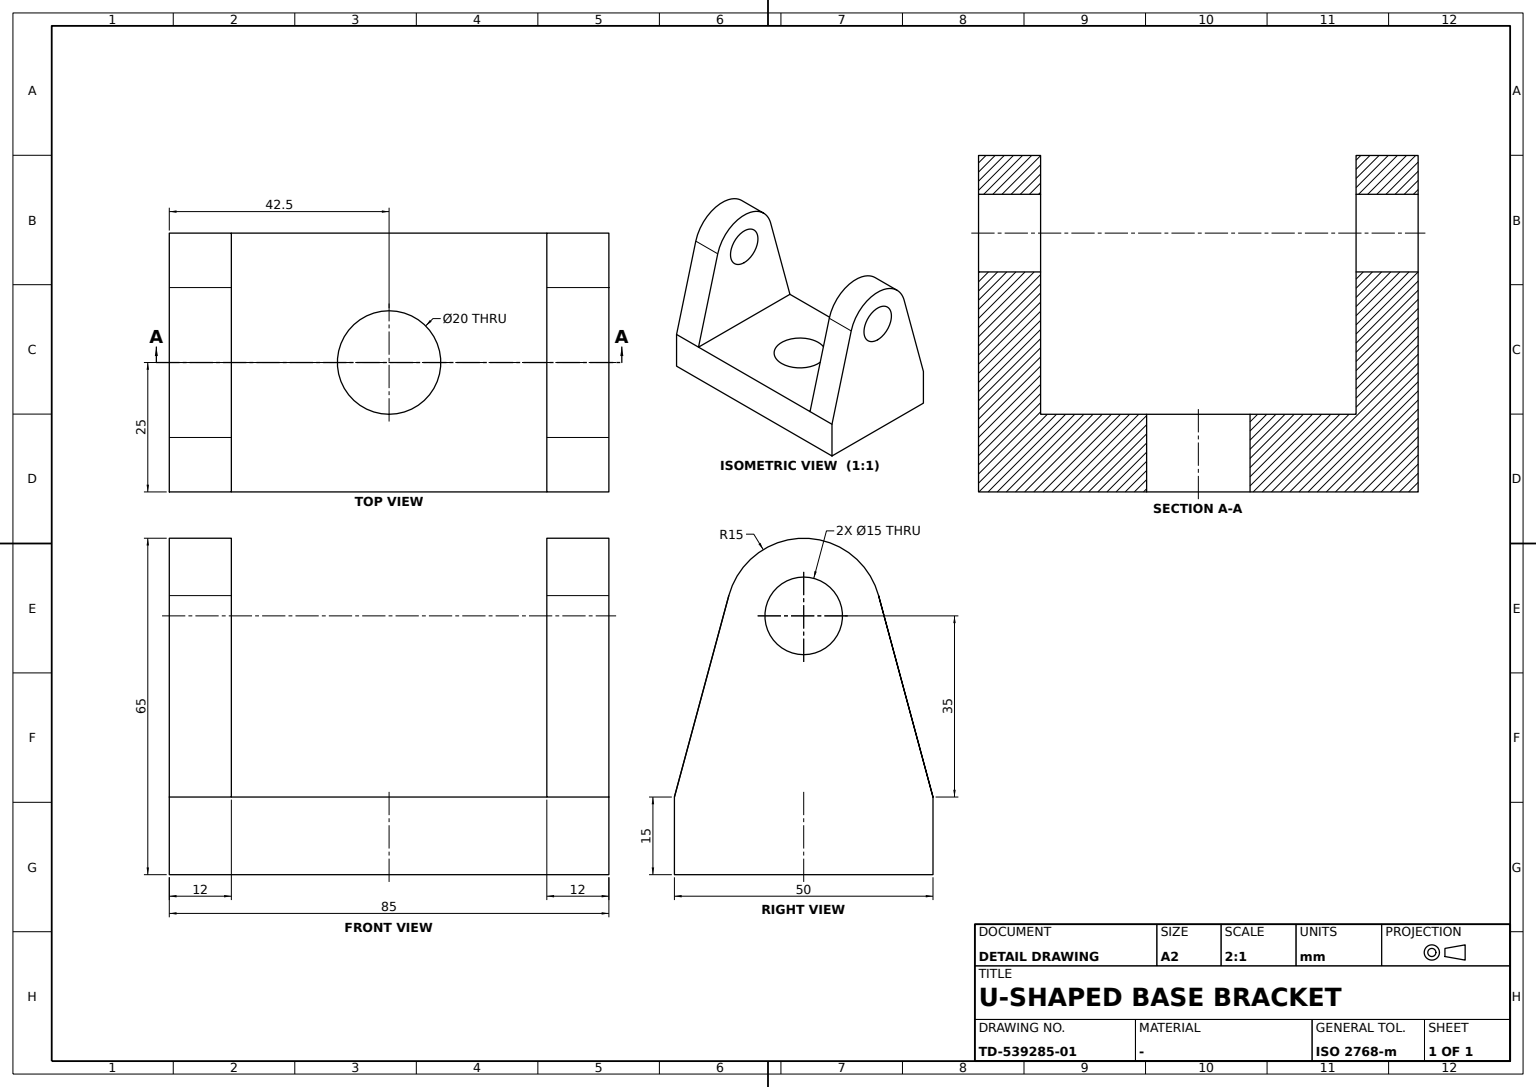
ISO-10303-21;
HEADER;
FILE_DESCRIPTION((''),'2;1');
FILE_NAME('','',(''),(''),'','','');
FILE_SCHEMA(('AUTOMOTIVE_DESIGN'));
ENDSEC;
DATA;
#1=APPLICATION_CONTEXT('');
#2=PRODUCT_CONTEXT('',#1,'mechanical');
#3=PRODUCT('','','',(#2));
#4=PRODUCT_DEFINITION_FORMATION('','',#3);
#5=PRODUCT_DEFINITION_CONTEXT('',#1,'design');
#6=PRODUCT_DEFINITION('','',#4,#5);
#7=PRODUCT_DEFINITION_SHAPE('','',#6);
#8=(LENGTH_UNIT()NAMED_UNIT(*)SI_UNIT(.MILLI.,.METRE.));
#9=(NAMED_UNIT(*)PLANE_ANGLE_UNIT()SI_UNIT($,.RADIAN.));
#10=(NAMED_UNIT(*)SI_UNIT($,.STERADIAN.)SOLID_ANGLE_UNIT());
#11=UNCERTAINTY_MEASURE_WITH_UNIT(LENGTH_MEASURE(0.005),#8,'distance_accuracy_value','');
#12=(GEOMETRIC_REPRESENTATION_CONTEXT(3)GLOBAL_UNCERTAINTY_ASSIGNED_CONTEXT((#11))GLOBAL_UNIT_ASSIGNED_CONTEXT((#8,#9,#10))REPRESENTATION_CONTEXT('',''));
#13=CARTESIAN_POINT('',(-14.480231,-42.5,53.91445));
#14=VERTEX_POINT('',#13);
#15=CARTESIAN_POINT('',(-14.480231,-30.5,53.91445));
#16=VERTEX_POINT('',#15);
#17=CARTESIAN_POINT('',(-14.480231,-36.5,53.91445));
#18=DIRECTION('',(0.,-1.,0.));
#19=VECTOR('',#18,1000.);
#20=LINE('',#17,#19);
#21=EDGE_CURVE('',#14,#16,#20,.F.);
#22=ORIENTED_EDGE('',*,*,#21,.T.);
#23=CARTESIAN_POINT('',(-25.,-30.5,15.));
#24=VERTEX_POINT('',#23);
#25=DIRECTION('',(-0.260963361,0.,-0.965348706));
#26=VECTOR('',#25,1000.);
#27=LINE('',#15,#26);
#28=EDGE_CURVE('',#16,#24,#27,.T.);
#29=ORIENTED_EDGE('',*,*,#28,.T.);
#30=CARTESIAN_POINT('',(-25.,-42.5,15.));
#31=VERTEX_POINT('',#30);
#32=DIRECTION('',(0.,1.,0.));
#33=VECTOR('',#32,1000.);
#34=LINE('',#30,#33);
#35=EDGE_CURVE('',#31,#24,#34,.T.);
#36=ORIENTED_EDGE('',*,*,#35,.F.);
#37=LINE('',#13,#26);
#38=EDGE_CURVE('',#14,#31,#37,.T.);
#39=ORIENTED_EDGE('',*,*,#38,.F.);
#40=EDGE_LOOP('',(#22,#29,#36,#39));
#41=FACE_BOUND('',#40,.T.);
#42=DIRECTION('',(0.965348706,0.,-0.260963361));
#43=AXIS2_PLACEMENT_3D('',#13,#42,#25);
#44=PLANE('',#43);
#45=ADVANCED_FACE('',(#41),#44,.F.);
#46=CARTESIAN_POINT('',(25.,30.5,15.));
#47=VERTEX_POINT('',#46);
#48=CARTESIAN_POINT('',(14.480231,30.5,53.91445));
#49=VERTEX_POINT('',#48);
#50=DIRECTION('',(-0.260963361,0.,0.965348706));
#51=VECTOR('',#50,1000.);
#52=LINE('',#46,#51);
#53=EDGE_CURVE('',#47,#49,#52,.T.);
#54=ORIENTED_EDGE('',*,*,#53,.T.);
#55=CARTESIAN_POINT('',(-14.480231,30.5,53.91445));
#56=VERTEX_POINT('',#55);
#57=CARTESIAN_POINT('',(0.,30.5,50.));
#58=DIRECTION('',(0.,0.,-1.));
#59=AXIS2_PLACEMENT_3D('',#57,#18,#58);
#60=CIRCLE('',#59,15.);
#61=EDGE_CURVE('',#49,#56,#60,.T.);
#62=ORIENTED_EDGE('',*,*,#61,.T.);
#63=CARTESIAN_POINT('',(-25.,30.5,15.));
#64=VERTEX_POINT('',#63);
#65=LINE('',#55,#26);
#66=EDGE_CURVE('',#56,#64,#65,.T.);
#67=ORIENTED_EDGE('',*,*,#66,.T.);
#68=CARTESIAN_POINT('',(0.,30.5,15.));
#69=DIRECTION('',(1.,0.,0.));
#70=VECTOR('',#69,1000.);
#71=LINE('',#68,#70);
#72=EDGE_CURVE('',#64,#47,#71,.T.);
#73=ORIENTED_EDGE('',*,*,#72,.T.);
#74=EDGE_LOOP('',(#54,#62,#67,#73));
#75=FACE_BOUND('',#74,.T.);
#76=CARTESIAN_POINT('',(0.,30.5,42.5));
#77=VERTEX_POINT('',#76);
#78=CIRCLE('',#59,7.5);
#79=EDGE_CURVE('',#77,#77,#78,.T.);
#80=ORIENTED_EDGE('',*,*,#79,.F.);
#81=EDGE_LOOP('',(#80));
#82=FACE_BOUND('',#81,.T.);
#83=CARTESIAN_POINT('',(0.,30.5,0.));
#84=AXIS2_PLACEMENT_3D('',#83,#18,#69);
#85=PLANE('',#84);
#86=ADVANCED_FACE('',(#75,#82),#85,.T.);
#87=CARTESIAN_POINT('',(25.,-30.5,15.));
#88=VERTEX_POINT('',#87);
#89=CARTESIAN_POINT('',(14.480231,-30.5,53.91445));
#90=VERTEX_POINT('',#89);
#91=LINE('',#87,#51);
#92=EDGE_CURVE('',#88,#90,#91,.T.);
#93=ORIENTED_EDGE('',*,*,#92,.F.);
#94=CARTESIAN_POINT('',(0.,-30.5,15.));
#95=LINE('',#94,#70);
#96=EDGE_CURVE('',#24,#88,#95,.T.);
#97=ORIENTED_EDGE('',*,*,#96,.F.);
#98=ORIENTED_EDGE('',*,*,#28,.F.);
#99=CARTESIAN_POINT('',(0.,-30.5,50.));
#100=AXIS2_PLACEMENT_3D('',#99,#18,#58);
#101=CIRCLE('',#100,15.);
#102=EDGE_CURVE('',#90,#16,#101,.T.);
#103=ORIENTED_EDGE('',*,*,#102,.F.);
#104=EDGE_LOOP('',(#93,#97,#98,#103));
#105=FACE_BOUND('',#104,.T.);
#106=CARTESIAN_POINT('',(0.,-30.5,42.5));
#107=VERTEX_POINT('',#106);
#108=CIRCLE('',#100,7.5);
#109=EDGE_CURVE('',#107,#107,#108,.T.);
#110=ORIENTED_EDGE('',*,*,#109,.T.);
#111=EDGE_LOOP('',(#110));
#112=FACE_BOUND('',#111,.T.);
#113=CARTESIAN_POINT('',(0.,-30.5,0.));
#114=AXIS2_PLACEMENT_3D('',#113,#18,#69);
#115=PLANE('',#114);
#116=ADVANCED_FACE('',(#105,#112),#115,.F.);
#117=CARTESIAN_POINT('',(-14.480231,42.5,53.91445));
#118=VERTEX_POINT('',#117);
#119=CARTESIAN_POINT('',(-25.,42.5,15.));
#120=VERTEX_POINT('',#119);
#121=LINE('',#117,#26);
#122=EDGE_CURVE('',#118,#120,#121,.T.);
#123=ORIENTED_EDGE('',*,*,#122,.T.);
#124=EDGE_CURVE('',#64,#120,#34,.T.);
#125=ORIENTED_EDGE('',*,*,#124,.F.);
#126=ORIENTED_EDGE('',*,*,#66,.F.);
#127=EDGE_CURVE('',#56,#118,#20,.F.);
#128=ORIENTED_EDGE('',*,*,#127,.T.);
#129=EDGE_LOOP('',(#123,#125,#126,#128));
#130=FACE_BOUND('',#129,.T.);
#131=ADVANCED_FACE('',(#130),#44,.F.);
#132=CARTESIAN_POINT('',(0.,-42.5,42.5));
#133=VERTEX_POINT('',#132);
#134=CARTESIAN_POINT('',(0.,-42.5,50.));
#135=AXIS2_PLACEMENT_3D('',#134,#18,#58);
#136=CIRCLE('',#135,7.5);
#137=EDGE_CURVE('',#133,#133,#136,.T.);
#138=ORIENTED_EDGE('',*,*,#137,.F.);
#139=EDGE_LOOP('',(#138));
#140=FACE_BOUND('',#139,.T.);
#141=CARTESIAN_POINT('',(25.,-42.5,15.));
#142=VERTEX_POINT('',#141);
#143=CARTESIAN_POINT('',(14.480231,-42.5,53.91445));
#144=VERTEX_POINT('',#143);
#145=LINE('',#141,#51);
#146=EDGE_CURVE('',#142,#144,#145,.T.);
#147=ORIENTED_EDGE('',*,*,#146,.T.);
#148=CIRCLE('',#135,15.);
#149=EDGE_CURVE('',#144,#14,#148,.T.);
#150=ORIENTED_EDGE('',*,*,#149,.T.);
#151=ORIENTED_EDGE('',*,*,#38,.T.);
#152=CARTESIAN_POINT('',(-25.,-42.5,0.));
#153=VERTEX_POINT('',#152);
#154=DIRECTION('',(0.,0.,1.));
#155=VECTOR('',#154,1000.);
#156=LINE('',#152,#155);
#157=EDGE_CURVE('',#153,#31,#156,.T.);
#158=ORIENTED_EDGE('',*,*,#157,.F.);
#159=CARTESIAN_POINT('',(25.,-42.5,0.));
#160=VERTEX_POINT('',#159);
#161=CARTESIAN_POINT('',(0.,-42.5,0.));
#162=LINE('',#161,#70);
#163=EDGE_CURVE('',#153,#160,#162,.T.);
#164=ORIENTED_EDGE('',*,*,#163,.T.);
#165=LINE('',#159,#155);
#166=EDGE_CURVE('',#160,#142,#165,.T.);
#167=ORIENTED_EDGE('',*,*,#166,.T.);
#168=EDGE_LOOP('',(#147,#150,#151,#158,#164,#167));
#169=FACE_BOUND('',#168,.T.);
#170=AXIS2_PLACEMENT_3D('',#152,#18,#69);
#171=PLANE('',#170);
#172=ADVANCED_FACE('',(#140,#169),#171,.T.);
#173=ORIENTED_EDGE('',*,*,#127,.F.);
#174=ORIENTED_EDGE('',*,*,#61,.F.);
#175=CARTESIAN_POINT('',(14.480231,42.5,53.91445));
#176=VERTEX_POINT('',#175);
#177=CARTESIAN_POINT('',(14.480231,-36.5,53.91445));
#178=LINE('',#177,#19);
#179=EDGE_CURVE('',#49,#176,#178,.F.);
#180=ORIENTED_EDGE('',*,*,#179,.T.);
#181=CARTESIAN_POINT('',(0.,42.5,50.));
#182=AXIS2_PLACEMENT_3D('',#181,#18,#58);
#183=CIRCLE('',#182,15.);
#184=EDGE_CURVE('',#176,#118,#183,.T.);
#185=ORIENTED_EDGE('',*,*,#184,.T.);
#186=EDGE_LOOP('',(#173,#174,#180,#185));
#187=FACE_BOUND('',#186,.T.);
#188=CARTESIAN_POINT('',(0.,-36.5,50.));
#189=AXIS2_PLACEMENT_3D('',#188,#18,#69);
#190=CYLINDRICAL_SURFACE('',#189,15.);
#191=ADVANCED_FACE('',(#187),#190,.T.);
#192=ORIENTED_EDGE('',*,*,#92,.T.);
#193=EDGE_CURVE('',#144,#90,#178,.F.);
#194=ORIENTED_EDGE('',*,*,#193,.F.);
#195=ORIENTED_EDGE('',*,*,#146,.F.);
#196=LINE('',#141,#33);
#197=EDGE_CURVE('',#142,#88,#196,.T.);
#198=ORIENTED_EDGE('',*,*,#197,.T.);
#199=EDGE_LOOP('',(#192,#194,#195,#198));
#200=FACE_BOUND('',#199,.T.);
#201=DIRECTION('',(-0.965348706,0.,-0.260963361));
#202=AXIS2_PLACEMENT_3D('',#141,#201,#50);
#203=PLANE('',#202);
#204=ADVANCED_FACE('',(#200),#203,.F.);
#205=CARTESIAN_POINT('',(-25.,0.,15.));
#206=LINE('',#205,#33);
#207=EDGE_CURVE('',#24,#64,#206,.T.);
#208=ORIENTED_EDGE('',*,*,#207,.F.);
#209=ORIENTED_EDGE('',*,*,#96,.T.);
#210=CARTESIAN_POINT('',(25.,0.,15.));
#211=LINE('',#210,#19);
#212=EDGE_CURVE('',#47,#88,#211,.T.);
#213=ORIENTED_EDGE('',*,*,#212,.F.);
#214=ORIENTED_EDGE('',*,*,#72,.F.);
#215=EDGE_LOOP('',(#208,#209,#213,#214));
#216=FACE_BOUND('',#215,.T.);
#217=CARTESIAN_POINT('',(10.,0.,15.));
#218=VERTEX_POINT('',#217);
#219=CARTESIAN_POINT('',(0.,0.,15.));
#220=AXIS2_PLACEMENT_3D('',#219,#154,#69);
#221=CIRCLE('',#220,10.);
#222=EDGE_CURVE('',#218,#218,#221,.T.);
#223=ORIENTED_EDGE('',*,*,#222,.F.);
#224=EDGE_LOOP('',(#223));
#225=FACE_BOUND('',#224,.T.);
#226=AXIS2_PLACEMENT_3D('',#219,#154,#32);
#227=PLANE('',#226);
#228=ADVANCED_FACE('',(#216,#225),#227,.T.);
#229=CARTESIAN_POINT('',(10.,0.,0.));
#230=VERTEX_POINT('',#229);
#231=CARTESIAN_POINT('',(0.,0.,0.));
#232=AXIS2_PLACEMENT_3D('',#231,#154,#69);
#233=CIRCLE('',#232,10.);
#234=EDGE_CURVE('',#230,#230,#233,.T.);
#235=ORIENTED_EDGE('',*,*,#234,.F.);
#236=EDGE_LOOP('',(#235));
#237=FACE_BOUND('',#236,.T.);
#238=ORIENTED_EDGE('',*,*,#222,.T.);
#239=EDGE_LOOP('',(#238));
#240=FACE_BOUND('',#239,.T.);
#241=CARTESIAN_POINT('',(0.,0.,7.5));
#242=AXIS2_PLACEMENT_3D('',#241,#154,#32);
#243=CYLINDRICAL_SURFACE('',#242,10.);
#244=ADVANCED_FACE('',(#237,#240),#243,.F.);
#245=ORIENTED_EDGE('',*,*,#79,.T.);
#246=EDGE_LOOP('',(#245));
#247=FACE_BOUND('',#246,.T.);
#248=CARTESIAN_POINT('',(0.,42.5,42.5));
#249=VERTEX_POINT('',#248);
#250=CIRCLE('',#182,7.5);
#251=EDGE_CURVE('',#249,#249,#250,.T.);
#252=ORIENTED_EDGE('',*,*,#251,.F.);
#253=EDGE_LOOP('',(#252));
#254=FACE_BOUND('',#253,.T.);
#255=CYLINDRICAL_SURFACE('',#189,7.5);
#256=ADVANCED_FACE('',(#247,#254),#255,.F.);
#257=CARTESIAN_POINT('',(25.,42.5,0.));
#258=VERTEX_POINT('',#257);
#259=CARTESIAN_POINT('',(25.,0.,0.));
#260=LINE('',#259,#19);
#261=EDGE_CURVE('',#258,#160,#260,.T.);
#262=ORIENTED_EDGE('',*,*,#261,.T.);
#263=ORIENTED_EDGE('',*,*,#163,.F.);
#264=CARTESIAN_POINT('',(-25.,42.5,0.));
#265=VERTEX_POINT('',#264);
#266=CARTESIAN_POINT('',(-25.,0.,0.));
#267=LINE('',#266,#33);
#268=EDGE_CURVE('',#153,#265,#267,.T.);
#269=ORIENTED_EDGE('',*,*,#268,.T.);
#270=DIRECTION('',(-1.,0.,0.));
#271=VECTOR('',#270,1000.);
#272=LINE('',#264,#271);
#273=EDGE_CURVE('',#258,#265,#272,.T.);
#274=ORIENTED_EDGE('',*,*,#273,.F.);
#275=EDGE_LOOP('',(#262,#263,#269,#274));
#276=FACE_BOUND('',#275,.T.);
#277=ORIENTED_EDGE('',*,*,#234,.T.);
#278=EDGE_LOOP('',(#277));
#279=FACE_BOUND('',#278,.T.);
#280=AXIS2_PLACEMENT_3D('',#231,#154,#32);
#281=PLANE('',#280);
#282=ADVANCED_FACE('',(#276,#279),#281,.F.);
#283=CARTESIAN_POINT('',(25.,42.5,15.));
#284=VERTEX_POINT('',#283);
#285=EDGE_CURVE('',#47,#284,#196,.T.);
#286=ORIENTED_EDGE('',*,*,#285,.T.);
#287=LINE('',#283,#51);
#288=EDGE_CURVE('',#284,#176,#287,.T.);
#289=ORIENTED_EDGE('',*,*,#288,.T.);
#290=ORIENTED_EDGE('',*,*,#179,.F.);
#291=ORIENTED_EDGE('',*,*,#53,.F.);
#292=EDGE_LOOP('',(#286,#289,#290,#291));
#293=FACE_BOUND('',#292,.T.);
#294=ADVANCED_FACE('',(#293),#203,.F.);
#295=LINE('',#264,#155);
#296=EDGE_CURVE('',#265,#120,#295,.T.);
#297=ORIENTED_EDGE('',*,*,#296,.F.);
#298=ORIENTED_EDGE('',*,*,#268,.F.);
#299=ORIENTED_EDGE('',*,*,#157,.T.);
#300=ORIENTED_EDGE('',*,*,#35,.T.);
#301=ORIENTED_EDGE('',*,*,#207,.T.);
#302=ORIENTED_EDGE('',*,*,#124,.T.);
#303=EDGE_LOOP('',(#297,#298,#299,#300,#301,#302));
#304=FACE_BOUND('',#303,.T.);
#305=AXIS2_PLACEMENT_3D('',#152,#69,#32);
#306=PLANE('',#305);
#307=ADVANCED_FACE('',(#304),#306,.F.);
#308=ORIENTED_EDGE('',*,*,#109,.F.);
#309=EDGE_LOOP('',(#308));
#310=FACE_BOUND('',#309,.T.);
#311=ORIENTED_EDGE('',*,*,#137,.T.);
#312=EDGE_LOOP('',(#311));
#313=FACE_BOUND('',#312,.T.);
#314=ADVANCED_FACE('',(#310,#313),#255,.F.);
#315=ORIENTED_EDGE('',*,*,#193,.T.);
#316=ORIENTED_EDGE('',*,*,#102,.T.);
#317=ORIENTED_EDGE('',*,*,#21,.F.);
#318=ORIENTED_EDGE('',*,*,#149,.F.);
#319=EDGE_LOOP('',(#315,#316,#317,#318));
#320=FACE_BOUND('',#319,.T.);
#321=ADVANCED_FACE('',(#320),#190,.T.);
#322=ORIENTED_EDGE('',*,*,#273,.T.);
#323=ORIENTED_EDGE('',*,*,#296,.T.);
#324=ORIENTED_EDGE('',*,*,#122,.F.);
#325=ORIENTED_EDGE('',*,*,#184,.F.);
#326=ORIENTED_EDGE('',*,*,#288,.F.);
#327=LINE('',#257,#155);
#328=EDGE_CURVE('',#258,#284,#327,.T.);
#329=ORIENTED_EDGE('',*,*,#328,.F.);
#330=EDGE_LOOP('',(#322,#323,#324,#325,#326,#329));
#331=FACE_BOUND('',#330,.T.);
#332=ORIENTED_EDGE('',*,*,#251,.T.);
#333=EDGE_LOOP('',(#332));
#334=FACE_BOUND('',#333,.T.);
#335=AXIS2_PLACEMENT_3D('',#264,#18,#69);
#336=PLANE('',#335);
#337=ADVANCED_FACE('',(#331,#334),#336,.F.);
#338=ORIENTED_EDGE('',*,*,#328,.T.);
#339=ORIENTED_EDGE('',*,*,#285,.F.);
#340=ORIENTED_EDGE('',*,*,#212,.T.);
#341=ORIENTED_EDGE('',*,*,#197,.F.);
#342=ORIENTED_EDGE('',*,*,#166,.F.);
#343=ORIENTED_EDGE('',*,*,#261,.F.);
#344=EDGE_LOOP('',(#338,#339,#340,#341,#342,#343));
#345=FACE_BOUND('',#344,.T.);
#346=AXIS2_PLACEMENT_3D('',#257,#270,#18);
#347=PLANE('',#346);
#348=ADVANCED_FACE('',(#345),#347,.F.);
#349=CLOSED_SHELL('',(#45,#86,#116,#131,#172,#191,#204,#228,#244,#256,#282,#294,#307,#314,#321,#337,#348));
#350=MANIFOLD_SOLID_BREP('',#349);
#351=ADVANCED_BREP_SHAPE_REPRESENTATION('',(#350),#12);
#352=SHAPE_DEFINITION_REPRESENTATION(#7,#351);
ENDSEC;
END-ISO-10303-21;
